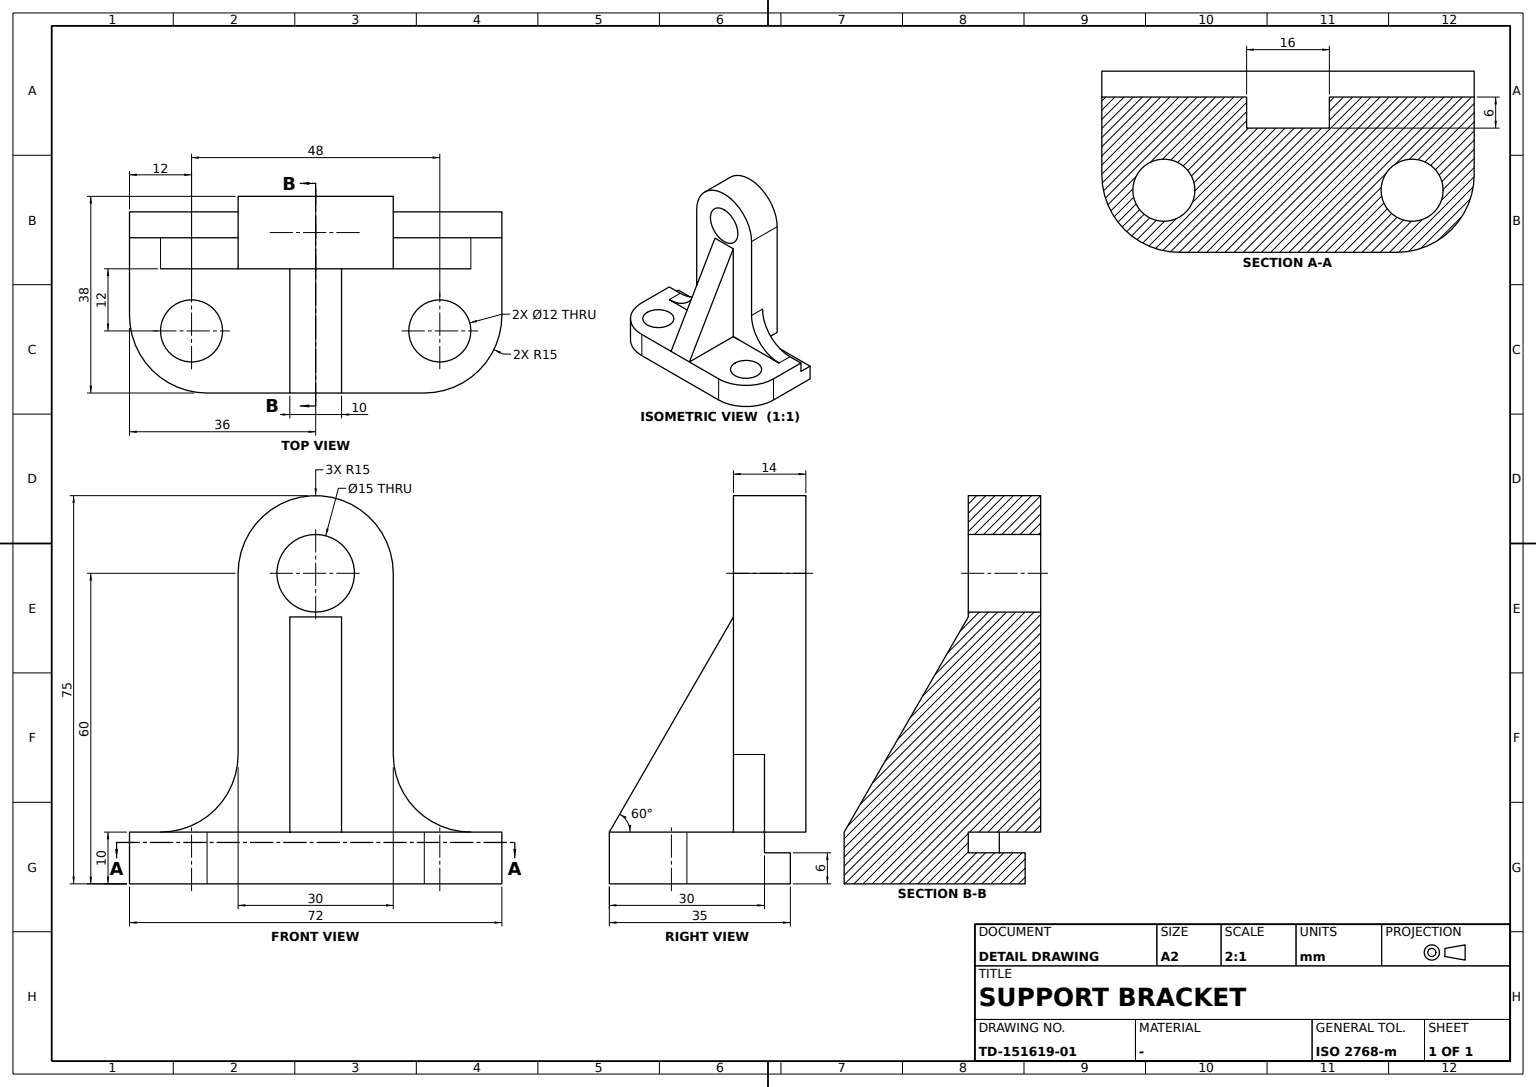
ISO-10303-21;
HEADER;
FILE_DESCRIPTION((''),'2;1');
FILE_NAME('','',(''),(''),'','','');
FILE_SCHEMA(('AUTOMOTIVE_DESIGN'));
ENDSEC;
DATA;
#1=APPLICATION_CONTEXT('');
#2=PRODUCT_CONTEXT('',#1,'mechanical');
#3=PRODUCT('','','',(#2));
#4=PRODUCT_DEFINITION_FORMATION('','',#3);
#5=PRODUCT_DEFINITION_CONTEXT('',#1,'design');
#6=PRODUCT_DEFINITION('','',#4,#5);
#7=PRODUCT_DEFINITION_SHAPE('','',#6);
#8=(LENGTH_UNIT()NAMED_UNIT(*)SI_UNIT(.MILLI.,.METRE.));
#9=(NAMED_UNIT(*)PLANE_ANGLE_UNIT()SI_UNIT($,.RADIAN.));
#10=(NAMED_UNIT(*)SI_UNIT($,.STERADIAN.)SOLID_ANGLE_UNIT());
#11=UNCERTAINTY_MEASURE_WITH_UNIT(LENGTH_MEASURE(0.005),#8,'distance_accuracy_value','');
#12=(GEOMETRIC_REPRESENTATION_CONTEXT(3)GLOBAL_UNCERTAINTY_ASSIGNED_CONTEXT((#11))GLOBAL_UNIT_ASSIGNED_CONTEXT((#8,#9,#10))REPRESENTATION_CONTEXT('',''));
#13=CARTESIAN_POINT('',(30.,6.5,5.));
#14=VERTEX_POINT('',#13);
#15=CARTESIAN_POINT('',(15.,6.5,20.));
#16=VERTEX_POINT('',#15);
#17=CARTESIAN_POINT('',(30.,6.5,20.));
#18=DIRECTION('',(0.,1.,0.));
#19=DIRECTION('',(0.,0.,1.));
#20=AXIS2_PLACEMENT_3D('',#17,#18,#19);
#21=CIRCLE('',#20,15.);
#22=EDGE_CURVE('',#14,#16,#21,.T.);
#23=ORIENTED_EDGE('',*,*,#22,.F.);
#24=CARTESIAN_POINT('',(30.,12.5,5.));
#25=VERTEX_POINT('',#24);
#26=CARTESIAN_POINT('',(30.,-0.1,5.));
#27=VECTOR('',#18,1000.);
#28=LINE('',#26,#27);
#29=EDGE_CURVE('',#14,#25,#28,.T.);
#30=ORIENTED_EDGE('',*,*,#29,.T.);
#31=CARTESIAN_POINT('',(15.,12.5,20.));
#32=VERTEX_POINT('',#31);
#33=CARTESIAN_POINT('',(30.,12.5,20.));
#34=DIRECTION('',(0.,-1.,0.));
#35=DIRECTION('',(0.,0.,-1.));
#36=AXIS2_PLACEMENT_3D('',#33,#34,#35);
#37=CIRCLE('',#36,15.);
#38=EDGE_CURVE('',#32,#25,#37,.T.);
#39=ORIENTED_EDGE('',*,*,#38,.F.);
#40=CARTESIAN_POINT('',(15.,-0.1,20.));
#41=LINE('',#40,#27);
#42=EDGE_CURVE('',#16,#32,#41,.T.);
#43=ORIENTED_EDGE('',*,*,#42,.F.);
#44=EDGE_LOOP('',(#23,#30,#39,#43));
#45=FACE_BOUND('',#44,.T.);
#46=CARTESIAN_POINT('',(30.,-0.1,20.));
#47=AXIS2_PLACEMENT_3D('',#46,#18,#35);
#48=CYLINDRICAL_SURFACE('',#47,15.);
#49=ADVANCED_FACE('',(#45),#48,.F.);
#50=CARTESIAN_POINT('',(-5.,6.5,46.569219));
#51=VERTEX_POINT('',#50);
#52=CARTESIAN_POINT('',(-5.,6.5,5.));
#53=VERTEX_POINT('',#52);
#54=CARTESIAN_POINT('',(-5.,6.5,0.));
#55=VECTOR('',#35,1000.);
#56=LINE('',#54,#55);
#57=EDGE_CURVE('',#51,#53,#56,.T.);
#58=ORIENTED_EDGE('',*,*,#57,.T.);
#59=CARTESIAN_POINT('',(-5.,-17.5,5.));
#60=VERTEX_POINT('',#59);
#61=CARTESIAN_POINT('',(-5.,0.,5.));
#62=LINE('',#61,#27);
#63=EDGE_CURVE('',#60,#53,#62,.T.);
#64=ORIENTED_EDGE('',*,*,#63,.F.);
#65=CARTESIAN_POINT('',(-5.,-15.290064,8.827722));
#66=DIRECTION('',(0.,0.5,0.866025404));
#67=VECTOR('',#66,1000.);
#68=LINE('',#65,#67);
#69=EDGE_CURVE('',#60,#51,#68,.T.);
#70=ORIENTED_EDGE('',*,*,#69,.T.);
#71=EDGE_LOOP('',(#58,#64,#70));
#72=FACE_BOUND('',#71,.T.);
#73=CARTESIAN_POINT('',(-5.,0.,0.));
#74=DIRECTION('',(1.,0.,0.));
#75=AXIS2_PLACEMENT_3D('',#73,#74,#18);
#76=PLANE('',#75);
#77=ADVANCED_FACE('',(#72),#76,.F.);
#78=CARTESIAN_POINT('',(-21.,-17.5,5.));
#79=VERTEX_POINT('',#78);
#80=CARTESIAN_POINT('',(-36.,-2.5,5.));
#81=VERTEX_POINT('',#80);
#82=CARTESIAN_POINT('',(-21.,-2.5,5.));
#83=DIRECTION('',(-1.,0.,0.));
#84=AXIS2_PLACEMENT_3D('',#82,#35,#83);
#85=CIRCLE('',#84,15.);
#86=EDGE_CURVE('',#79,#81,#85,.T.);
#87=ORIENTED_EDGE('',*,*,#86,.T.);
#88=CARTESIAN_POINT('',(-36.,-2.5,-5.));
#89=VERTEX_POINT('',#88);
#90=CARTESIAN_POINT('',(-36.,-2.5,0.));
#91=VECTOR('',#19,1000.);
#92=LINE('',#90,#91);
#93=EDGE_CURVE('',#89,#81,#92,.T.);
#94=ORIENTED_EDGE('',*,*,#93,.F.);
#95=CARTESIAN_POINT('',(-21.,-17.5,-5.));
#96=VERTEX_POINT('',#95);
#97=CARTESIAN_POINT('',(-21.,-2.5,-5.));
#98=AXIS2_PLACEMENT_3D('',#97,#19,#74);
#99=CIRCLE('',#98,15.);
#100=EDGE_CURVE('',#89,#96,#99,.T.);
#101=ORIENTED_EDGE('',*,*,#100,.T.);
#102=CARTESIAN_POINT('',(-21.,-17.5,0.));
#103=LINE('',#102,#91);
#104=EDGE_CURVE('',#96,#79,#103,.T.);
#105=ORIENTED_EDGE('',*,*,#104,.T.);
#106=EDGE_LOOP('',(#87,#94,#101,#105));
#107=FACE_BOUND('',#106,.T.);
#108=CARTESIAN_POINT('',(-21.,-2.5,0.));
#109=AXIS2_PLACEMENT_3D('',#108,#19,#83);
#110=CYLINDRICAL_SURFACE('',#109,15.);
#111=ADVANCED_FACE('',(#107),#110,.T.);
#112=CARTESIAN_POINT('',(15.,6.5,55.));
#113=VERTEX_POINT('',#112);
#114=CARTESIAN_POINT('',(15.,20.5,55.));
#115=VERTEX_POINT('',#114);
#116=CARTESIAN_POINT('',(15.,13.5,55.));
#117=LINE('',#116,#27);
#118=EDGE_CURVE('',#113,#115,#117,.T.);
#119=ORIENTED_EDGE('',*,*,#118,.F.);
#120=CARTESIAN_POINT('',(15.,6.5,0.));
#121=LINE('',#120,#55);
#122=EDGE_CURVE('',#113,#16,#121,.T.);
#123=ORIENTED_EDGE('',*,*,#122,.T.);
#124=ORIENTED_EDGE('',*,*,#42,.T.);
#125=CARTESIAN_POINT('',(15.,12.5,5.));
#126=VERTEX_POINT('',#125);
#127=CARTESIAN_POINT('',(15.,12.5,55.));
#128=LINE('',#127,#55);
#129=EDGE_CURVE('',#32,#126,#128,.T.);
#130=ORIENTED_EDGE('',*,*,#129,.T.);
#131=CARTESIAN_POINT('',(15.,20.5,5.));
#132=VERTEX_POINT('',#131);
#133=CARTESIAN_POINT('',(15.,6.5,5.));
#134=LINE('',#133,#27);
#135=EDGE_CURVE('',#126,#132,#134,.T.);
#136=ORIENTED_EDGE('',*,*,#135,.T.);
#137=CARTESIAN_POINT('',(15.,20.5,0.));
#138=LINE('',#137,#55);
#139=EDGE_CURVE('',#115,#132,#138,.T.);
#140=ORIENTED_EDGE('',*,*,#139,.F.);
#141=EDGE_LOOP('',(#119,#123,#124,#130,#136,#140));
#142=FACE_BOUND('',#141,.T.);
#143=AXIS2_PLACEMENT_3D('',#112,#74,#35);
#144=PLANE('',#143);
#145=ADVANCED_FACE('',(#142),#144,.T.);
#146=CARTESIAN_POINT('',(5.,-17.5,5.));
#147=VERTEX_POINT('',#146);
#148=CARTESIAN_POINT('',(5.,6.5,5.));
#149=VERTEX_POINT('',#148);
#150=CARTESIAN_POINT('',(5.,0.,5.));
#151=LINE('',#150,#27);
#152=EDGE_CURVE('',#147,#149,#151,.T.);
#153=ORIENTED_EDGE('',*,*,#152,.T.);
#154=CARTESIAN_POINT('',(5.,6.5,46.569219));
#155=VERTEX_POINT('',#154);
#156=CARTESIAN_POINT('',(5.,6.5,0.));
#157=LINE('',#156,#55);
#158=EDGE_CURVE('',#155,#149,#157,.T.);
#159=ORIENTED_EDGE('',*,*,#158,.F.);
#160=CARTESIAN_POINT('',(5.,-15.290064,8.827722));
#161=LINE('',#160,#67);
#162=EDGE_CURVE('',#147,#155,#161,.T.);
#163=ORIENTED_EDGE('',*,*,#162,.F.);
#164=EDGE_LOOP('',(#153,#159,#163));
#165=FACE_BOUND('',#164,.T.);
#166=CARTESIAN_POINT('',(5.,0.,0.));
#167=AXIS2_PLACEMENT_3D('',#166,#74,#18);
#168=PLANE('',#167);
#169=ADVANCED_FACE('',(#165),#168,.T.);
#170=ORIENTED_EDGE('',*,*,#139,.T.);
#171=CARTESIAN_POINT('',(-15.,20.5,5.));
#172=VERTEX_POINT('',#171);
#173=CARTESIAN_POINT('',(0.,20.5,5.));
#174=VECTOR('',#83,1000.);
#175=LINE('',#173,#174);
#176=EDGE_CURVE('',#132,#172,#175,.T.);
#177=ORIENTED_EDGE('',*,*,#176,.T.);
#178=CARTESIAN_POINT('',(-15.,20.5,55.));
#179=VERTEX_POINT('',#178);
#180=CARTESIAN_POINT('',(-15.,20.5,0.));
#181=LINE('',#180,#91);
#182=EDGE_CURVE('',#172,#179,#181,.T.);
#183=ORIENTED_EDGE('',*,*,#182,.T.);
#184=CARTESIAN_POINT('',(0.,20.5,55.));
#185=AXIS2_PLACEMENT_3D('',#184,#18,#19);
#186=CIRCLE('',#185,15.);
#187=EDGE_CURVE('',#179,#115,#186,.T.);
#188=ORIENTED_EDGE('',*,*,#187,.T.);
#189=EDGE_LOOP('',(#170,#177,#183,#188));
#190=FACE_BOUND('',#189,.T.);
#191=CARTESIAN_POINT('',(0.,20.5,62.5));
#192=VERTEX_POINT('',#191);
#193=CIRCLE('',#185,7.5);
#194=EDGE_CURVE('',#192,#192,#193,.T.);
#195=ORIENTED_EDGE('',*,*,#194,.F.);
#196=EDGE_LOOP('',(#195));
#197=FACE_BOUND('',#196,.T.);
#198=CARTESIAN_POINT('',(0.,20.5,0.));
#199=AXIS2_PLACEMENT_3D('',#198,#18,#83);
#200=PLANE('',#199);
#201=ADVANCED_FACE('',(#190,#197),#200,.T.);
#202=CARTESIAN_POINT('',(-18.,-5.5,-5.));
#203=VERTEX_POINT('',#202);
#204=CARTESIAN_POINT('',(-24.,-5.5,-5.));
#205=AXIS2_PLACEMENT_3D('',#204,#19,#74);
#206=CIRCLE('',#205,6.);
#207=EDGE_CURVE('',#203,#203,#206,.T.);
#208=ORIENTED_EDGE('',*,*,#207,.F.);
#209=EDGE_LOOP('',(#208));
#210=FACE_BOUND('',#209,.T.);
#211=CARTESIAN_POINT('',(-30.,-5.5,5.));
#212=VERTEX_POINT('',#211);
#213=CARTESIAN_POINT('',(-24.,-5.5,5.));
#214=AXIS2_PLACEMENT_3D('',#213,#35,#83);
#215=CIRCLE('',#214,6.);
#216=EDGE_CURVE('',#212,#212,#215,.F.);
#217=ORIENTED_EDGE('',*,*,#216,.T.);
#218=EDGE_LOOP('',(#217));
#219=FACE_BOUND('',#218,.T.);
#220=CARTESIAN_POINT('',(-24.,-5.5,-0.66));
#221=AXIS2_PLACEMENT_3D('',#220,#19,#34);
#222=CYLINDRICAL_SURFACE('',#221,6.);
#223=ADVANCED_FACE('',(#210,#219),#222,.F.);
#224=ORIENTED_EDGE('',*,*,#187,.F.);
#225=CARTESIAN_POINT('',(-15.,6.5,55.));
#226=VERTEX_POINT('',#225);
#227=CARTESIAN_POINT('',(-15.,13.5,55.));
#228=LINE('',#227,#27);
#229=EDGE_CURVE('',#226,#179,#228,.T.);
#230=ORIENTED_EDGE('',*,*,#229,.F.);
#231=CARTESIAN_POINT('',(0.,6.5,55.));
#232=AXIS2_PLACEMENT_3D('',#231,#18,#19);
#233=CIRCLE('',#232,15.);
#234=EDGE_CURVE('',#226,#113,#233,.T.);
#235=ORIENTED_EDGE('',*,*,#234,.T.);
#236=ORIENTED_EDGE('',*,*,#118,.T.);
#237=EDGE_LOOP('',(#224,#230,#235,#236));
#238=FACE_BOUND('',#237,.T.);
#239=CARTESIAN_POINT('',(0.,13.5,55.));
#240=AXIS2_PLACEMENT_3D('',#239,#18,#83);
#241=CYLINDRICAL_SURFACE('',#240,15.);
#242=ADVANCED_FACE('',(#238),#241,.T.);
#243=CARTESIAN_POINT('',(8.,6.5,1.));
#244=VERTEX_POINT('',#243);
#245=CARTESIAN_POINT('',(-8.,6.5,1.));
#246=VERTEX_POINT('',#245);
#247=CARTESIAN_POINT('',(0.,6.5,1.));
#248=LINE('',#247,#174);
#249=EDGE_CURVE('',#244,#246,#248,.T.);
#250=ORIENTED_EDGE('',*,*,#249,.T.);
#251=CARTESIAN_POINT('',(-8.,6.5,5.));
#252=VERTEX_POINT('',#251);
#253=LINE('',#245,#91);
#254=EDGE_CURVE('',#246,#252,#253,.T.);
#255=ORIENTED_EDGE('',*,*,#254,.T.);
#256=CARTESIAN_POINT('',(0.,6.5,5.));
#257=LINE('',#256,#174);
#258=EDGE_CURVE('',#149,#252,#257,.T.);
#259=ORIENTED_EDGE('',*,*,#258,.F.);
#260=CARTESIAN_POINT('',(8.,6.5,5.));
#261=VERTEX_POINT('',#260);
#262=EDGE_CURVE('',#261,#149,#257,.T.);
#263=ORIENTED_EDGE('',*,*,#262,.F.);
#264=LINE('',#260,#55);
#265=EDGE_CURVE('',#261,#244,#264,.T.);
#266=ORIENTED_EDGE('',*,*,#265,.T.);
#267=EDGE_LOOP('',(#250,#255,#259,#263,#266));
#268=FACE_BOUND('',#267,.T.);
#269=CARTESIAN_POINT('',(0.,6.5,0.));
#270=AXIS2_PLACEMENT_3D('',#269,#18,#83);
#271=PLANE('',#270);
#272=ADVANCED_FACE('',(#268),#271,.T.);
#273=CARTESIAN_POINT('',(36.,-2.5,5.));
#274=VERTEX_POINT('',#273);
#275=CARTESIAN_POINT('',(36.,12.5,5.));
#276=VERTEX_POINT('',#275);
#277=CARTESIAN_POINT('',(36.,0.,5.));
#278=LINE('',#277,#27);
#279=EDGE_CURVE('',#274,#276,#278,.T.);
#280=ORIENTED_EDGE('',*,*,#279,.T.);
#281=CARTESIAN_POINT('',(0.,12.5,5.));
#282=VECTOR('',#74,1000.);
#283=LINE('',#281,#282);
#284=EDGE_CURVE('',#25,#276,#283,.T.);
#285=ORIENTED_EDGE('',*,*,#284,.F.);
#286=ORIENTED_EDGE('',*,*,#29,.F.);
#287=EDGE_CURVE('',#14,#261,#257,.T.);
#288=ORIENTED_EDGE('',*,*,#287,.T.);
#289=ORIENTED_EDGE('',*,*,#262,.T.);
#290=ORIENTED_EDGE('',*,*,#152,.F.);
#291=CARTESIAN_POINT('',(21.,-17.5,5.));
#292=VERTEX_POINT('',#291);
#293=CARTESIAN_POINT('',(0.,-17.5,5.));
#294=LINE('',#293,#282);
#295=EDGE_CURVE('',#147,#292,#294,.T.);
#296=ORIENTED_EDGE('',*,*,#295,.T.);
#297=CARTESIAN_POINT('',(21.,-2.5,5.));
#298=AXIS2_PLACEMENT_3D('',#297,#35,#83);
#299=CIRCLE('',#298,15.);
#300=EDGE_CURVE('',#274,#292,#299,.T.);
#301=ORIENTED_EDGE('',*,*,#300,.F.);
#302=EDGE_LOOP('',(#280,#285,#286,#288,#289,#290,#296,#301));
#303=FACE_BOUND('',#302,.T.);
#304=CARTESIAN_POINT('',(18.,-5.5,5.));
#305=VERTEX_POINT('',#304);
#306=CARTESIAN_POINT('',(24.,-5.5,5.));
#307=AXIS2_PLACEMENT_3D('',#306,#35,#83);
#308=CIRCLE('',#307,6.);
#309=EDGE_CURVE('',#305,#305,#308,.F.);
#310=ORIENTED_EDGE('',*,*,#309,.F.);
#311=EDGE_LOOP('',(#310));
#312=FACE_BOUND('',#311,.T.);
#313=AXIS2_PLACEMENT_3D('',#293,#35,#18);
#314=PLANE('',#313);
#315=ADVANCED_FACE('',(#303,#312),#314,.F.);
#316=CARTESIAN_POINT('',(8.,12.5,1.));
#317=VERTEX_POINT('',#316);
#318=VECTOR('',#34,1000.);
#319=LINE('',#316,#318);
#320=EDGE_CURVE('',#317,#244,#319,.T.);
#321=ORIENTED_EDGE('',*,*,#320,.T.);
#322=ORIENTED_EDGE('',*,*,#265,.F.);
#323=CARTESIAN_POINT('',(8.,12.5,5.));
#324=VERTEX_POINT('',#323);
#325=LINE('',#323,#318);
#326=EDGE_CURVE('',#324,#261,#325,.T.);
#327=ORIENTED_EDGE('',*,*,#326,.F.);
#328=LINE('',#323,#55);
#329=EDGE_CURVE('',#324,#317,#328,.T.);
#330=ORIENTED_EDGE('',*,*,#329,.T.);
#331=EDGE_LOOP('',(#321,#322,#327,#330));
#332=FACE_BOUND('',#331,.T.);
#333=AXIS2_PLACEMENT_3D('',#323,#83,#35);
#334=PLANE('',#333);
#335=ADVANCED_FACE('',(#332),#334,.T.);
#336=ORIENTED_EDGE('',*,*,#194,.T.);
#337=EDGE_LOOP('',(#336));
#338=FACE_BOUND('',#337,.T.);
#339=CARTESIAN_POINT('',(0.,6.5,62.5));
#340=VERTEX_POINT('',#339);
#341=CIRCLE('',#232,7.5);
#342=EDGE_CURVE('',#340,#340,#341,.T.);
#343=ORIENTED_EDGE('',*,*,#342,.F.);
#344=EDGE_LOOP('',(#343));
#345=FACE_BOUND('',#344,.T.);
#346=CYLINDRICAL_SURFACE('',#240,7.5);
#347=ADVANCED_FACE('',(#338,#345),#346,.F.);
#348=CARTESIAN_POINT('',(-8.,12.5,1.));
#349=VERTEX_POINT('',#348);
#350=LINE('',#348,#318);
#351=EDGE_CURVE('',#349,#246,#350,.T.);
#352=ORIENTED_EDGE('',*,*,#351,.T.);
#353=ORIENTED_EDGE('',*,*,#249,.F.);
#354=ORIENTED_EDGE('',*,*,#320,.F.);
#355=CARTESIAN_POINT('',(36.,12.5,1.));
#356=VERTEX_POINT('',#355);
#357=CARTESIAN_POINT('',(0.,12.5,1.));
#358=LINE('',#357,#282);
#359=EDGE_CURVE('',#317,#356,#358,.T.);
#360=ORIENTED_EDGE('',*,*,#359,.T.);
#361=CARTESIAN_POINT('',(36.,17.5,1.));
#362=VERTEX_POINT('',#361);
#363=CARTESIAN_POINT('',(36.,0.,1.));
#364=LINE('',#363,#27);
#365=EDGE_CURVE('',#356,#362,#364,.T.);
#366=ORIENTED_EDGE('',*,*,#365,.T.);
#367=CARTESIAN_POINT('',(-36.,17.5,1.));
#368=VERTEX_POINT('',#367);
#369=CARTESIAN_POINT('',(0.,17.5,1.));
#370=LINE('',#369,#282);
#371=EDGE_CURVE('',#368,#362,#370,.T.);
#372=ORIENTED_EDGE('',*,*,#371,.F.);
#373=CARTESIAN_POINT('',(-36.,12.5,1.));
#374=VERTEX_POINT('',#373);
#375=CARTESIAN_POINT('',(-36.,0.,1.));
#376=LINE('',#375,#27);
#377=EDGE_CURVE('',#374,#368,#376,.T.);
#378=ORIENTED_EDGE('',*,*,#377,.F.);
#379=EDGE_CURVE('',#374,#349,#358,.T.);
#380=ORIENTED_EDGE('',*,*,#379,.T.);
#381=EDGE_LOOP('',(#352,#353,#354,#360,#366,#372,#378,#380));
#382=FACE_BOUND('',#381,.T.);
#383=AXIS2_PLACEMENT_3D('',#357,#35,#18);
#384=PLANE('',#383);
#385=ADVANCED_FACE('',(#382),#384,.F.);
#386=CARTESIAN_POINT('',(30.,-5.5,-5.));
#387=VERTEX_POINT('',#386);
#388=CARTESIAN_POINT('',(24.,-5.5,-5.));
#389=AXIS2_PLACEMENT_3D('',#388,#19,#74);
#390=CIRCLE('',#389,6.);
#391=EDGE_CURVE('',#387,#387,#390,.T.);
#392=ORIENTED_EDGE('',*,*,#391,.F.);
#393=EDGE_LOOP('',(#392));
#394=FACE_BOUND('',#393,.T.);
#395=ORIENTED_EDGE('',*,*,#309,.T.);
#396=EDGE_LOOP('',(#395));
#397=FACE_BOUND('',#396,.T.);
#398=CARTESIAN_POINT('',(24.,-5.5,-0.66));
#399=AXIS2_PLACEMENT_3D('',#398,#19,#34);
#400=CYLINDRICAL_SURFACE('',#399,6.);
#401=ADVANCED_FACE('',(#394,#397),#400,.F.);
#402=ORIENTED_EDGE('',*,*,#229,.T.);
#403=ORIENTED_EDGE('',*,*,#182,.F.);
#404=CARTESIAN_POINT('',(-15.,12.5,5.));
#405=VERTEX_POINT('',#404);
#406=CARTESIAN_POINT('',(-15.,-17.5,5.));
#407=LINE('',#406,#27);
#408=EDGE_CURVE('',#405,#172,#407,.T.);
#409=ORIENTED_EDGE('',*,*,#408,.F.);
#410=CARTESIAN_POINT('',(-15.,12.5,20.));
#411=VERTEX_POINT('',#410);
#412=LINE('',#404,#91);
#413=EDGE_CURVE('',#405,#411,#412,.T.);
#414=ORIENTED_EDGE('',*,*,#413,.T.);
#415=CARTESIAN_POINT('',(-15.,6.5,20.));
#416=VERTEX_POINT('',#415);
#417=CARTESIAN_POINT('',(-15.,-0.1,20.));
#418=LINE('',#417,#318);
#419=EDGE_CURVE('',#411,#416,#418,.T.);
#420=ORIENTED_EDGE('',*,*,#419,.T.);
#421=CARTESIAN_POINT('',(-15.,6.5,0.));
#422=LINE('',#421,#91);
#423=EDGE_CURVE('',#416,#226,#422,.T.);
#424=ORIENTED_EDGE('',*,*,#423,.T.);
#425=EDGE_LOOP('',(#402,#403,#409,#414,#420,#424));
#426=FACE_BOUND('',#425,.T.);
#427=CARTESIAN_POINT('',(-15.,6.5,5.));
#428=AXIS2_PLACEMENT_3D('',#427,#83,#19);
#429=PLANE('',#428);
#430=ADVANCED_FACE('',(#426),#429,.T.);
#431=ORIENTED_EDGE('',*,*,#162,.T.);
#432=CARTESIAN_POINT('',(0.,6.5,46.569219));
#433=LINE('',#432,#282);
#434=EDGE_CURVE('',#51,#155,#433,.T.);
#435=ORIENTED_EDGE('',*,*,#434,.F.);
#436=ORIENTED_EDGE('',*,*,#69,.F.);
#437=EDGE_CURVE('',#60,#147,#294,.T.);
#438=ORIENTED_EDGE('',*,*,#437,.T.);
#439=EDGE_LOOP('',(#431,#435,#436,#438));
#440=FACE_BOUND('',#439,.T.);
#441=DIRECTION('',(0.,0.866025404,-0.5));
#442=AXIS2_PLACEMENT_3D('',#293,#441,#66);
#443=PLANE('',#442);
#444=ADVANCED_FACE('',(#440),#443,.F.);
#445=ORIENTED_EDGE('',*,*,#300,.T.);
#446=CARTESIAN_POINT('',(21.,-17.5,-5.));
#447=VERTEX_POINT('',#446);
#448=CARTESIAN_POINT('',(21.,-17.5,0.));
#449=LINE('',#448,#91);
#450=EDGE_CURVE('',#447,#292,#449,.T.);
#451=ORIENTED_EDGE('',*,*,#450,.F.);
#452=CARTESIAN_POINT('',(36.,-2.5,-5.));
#453=VERTEX_POINT('',#452);
#454=CARTESIAN_POINT('',(21.,-2.5,-5.));
#455=AXIS2_PLACEMENT_3D('',#454,#19,#74);
#456=CIRCLE('',#455,15.);
#457=EDGE_CURVE('',#447,#453,#456,.T.);
#458=ORIENTED_EDGE('',*,*,#457,.T.);
#459=CARTESIAN_POINT('',(36.,-2.5,0.));
#460=LINE('',#459,#91);
#461=EDGE_CURVE('',#453,#274,#460,.T.);
#462=ORIENTED_EDGE('',*,*,#461,.T.);
#463=EDGE_LOOP('',(#445,#451,#458,#462));
#464=FACE_BOUND('',#463,.T.);
#465=CARTESIAN_POINT('',(21.,-2.5,0.));
#466=AXIS2_PLACEMENT_3D('',#465,#19,#34);
#467=CYLINDRICAL_SURFACE('',#466,15.);
#468=ADVANCED_FACE('',(#464),#467,.T.);
#469=ORIENTED_EDGE('',*,*,#329,.F.);
#470=EDGE_CURVE('',#324,#126,#283,.T.);
#471=ORIENTED_EDGE('',*,*,#470,.T.);
#472=ORIENTED_EDGE('',*,*,#129,.F.);
#473=ORIENTED_EDGE('',*,*,#38,.T.);
#474=ORIENTED_EDGE('',*,*,#284,.T.);
#475=CARTESIAN_POINT('',(36.,12.5,0.));
#476=LINE('',#475,#55);
#477=EDGE_CURVE('',#276,#356,#476,.T.);
#478=ORIENTED_EDGE('',*,*,#477,.T.);
#479=ORIENTED_EDGE('',*,*,#359,.F.);
#480=EDGE_LOOP('',(#469,#471,#472,#473,#474,#478,#479));
#481=FACE_BOUND('',#480,.T.);
#482=AXIS2_PLACEMENT_3D('',#281,#34,#35);
#483=PLANE('',#482);
#484=ADVANCED_FACE('',(#481),#483,.F.);
#485=ORIENTED_EDGE('',*,*,#461,.F.);
#486=CARTESIAN_POINT('',(36.,17.5,-5.));
#487=VERTEX_POINT('',#486);
#488=CARTESIAN_POINT('',(36.,0.,-5.));
#489=LINE('',#488,#318);
#490=EDGE_CURVE('',#487,#453,#489,.T.);
#491=ORIENTED_EDGE('',*,*,#490,.F.);
#492=CARTESIAN_POINT('',(36.,17.5,0.));
#493=LINE('',#492,#55);
#494=EDGE_CURVE('',#362,#487,#493,.T.);
#495=ORIENTED_EDGE('',*,*,#494,.F.);
#496=ORIENTED_EDGE('',*,*,#365,.F.);
#497=ORIENTED_EDGE('',*,*,#477,.F.);
#498=ORIENTED_EDGE('',*,*,#279,.F.);
#499=EDGE_LOOP('',(#485,#491,#495,#496,#497,#498));
#500=FACE_BOUND('',#499,.T.);
#501=CARTESIAN_POINT('',(36.,0.,0.));
#502=AXIS2_PLACEMENT_3D('',#501,#74,#18);
#503=PLANE('',#502);
#504=ADVANCED_FACE('',(#500),#503,.T.);
#505=CARTESIAN_POINT('',(-36.,17.5,-5.));
#506=VERTEX_POINT('',#505);
#507=CARTESIAN_POINT('',(-36.,0.,-5.));
#508=LINE('',#507,#318);
#509=EDGE_CURVE('',#506,#89,#508,.T.);
#510=ORIENTED_EDGE('',*,*,#509,.T.);
#511=ORIENTED_EDGE('',*,*,#93,.T.);
#512=CARTESIAN_POINT('',(-36.,12.5,5.));
#513=VERTEX_POINT('',#512);
#514=CARTESIAN_POINT('',(-36.,0.,5.));
#515=LINE('',#514,#27);
#516=EDGE_CURVE('',#81,#513,#515,.T.);
#517=ORIENTED_EDGE('',*,*,#516,.T.);
#518=CARTESIAN_POINT('',(-36.,12.5,0.));
#519=LINE('',#518,#55);
#520=EDGE_CURVE('',#513,#374,#519,.T.);
#521=ORIENTED_EDGE('',*,*,#520,.T.);
#522=ORIENTED_EDGE('',*,*,#377,.T.);
#523=CARTESIAN_POINT('',(-36.,17.5,0.));
#524=LINE('',#523,#55);
#525=EDGE_CURVE('',#368,#506,#524,.T.);
#526=ORIENTED_EDGE('',*,*,#525,.T.);
#527=EDGE_LOOP('',(#510,#511,#517,#521,#522,#526));
#528=FACE_BOUND('',#527,.T.);
#529=CARTESIAN_POINT('',(-36.,0.,0.));
#530=AXIS2_PLACEMENT_3D('',#529,#74,#18);
#531=PLANE('',#530);
#532=ADVANCED_FACE('',(#528),#531,.F.);
#533=ORIENTED_EDGE('',*,*,#494,.T.);
#534=CARTESIAN_POINT('',(0.,17.5,-5.));
#535=LINE('',#534,#282);
#536=EDGE_CURVE('',#506,#487,#535,.T.);
#537=ORIENTED_EDGE('',*,*,#536,.F.);
#538=ORIENTED_EDGE('',*,*,#525,.F.);
#539=ORIENTED_EDGE('',*,*,#371,.T.);
#540=EDGE_LOOP('',(#533,#537,#538,#539));
#541=FACE_BOUND('',#540,.T.);
#542=AXIS2_PLACEMENT_3D('',#369,#34,#35);
#543=PLANE('',#542);
#544=ADVANCED_FACE('',(#541),#543,.F.);
#545=ORIENTED_EDGE('',*,*,#86,.F.);
#546=EDGE_CURVE('',#79,#60,#294,.T.);
#547=ORIENTED_EDGE('',*,*,#546,.T.);
#548=ORIENTED_EDGE('',*,*,#63,.T.);
#549=CARTESIAN_POINT('',(-30.,6.5,5.));
#550=VERTEX_POINT('',#549);
#551=EDGE_CURVE('',#53,#550,#257,.T.);
#552=ORIENTED_EDGE('',*,*,#551,.T.);
#553=CARTESIAN_POINT('',(-30.,12.5,5.));
#554=VERTEX_POINT('',#553);
#555=CARTESIAN_POINT('',(-30.,-0.1,5.));
#556=LINE('',#555,#318);
#557=EDGE_CURVE('',#554,#550,#556,.T.);
#558=ORIENTED_EDGE('',*,*,#557,.F.);
#559=EDGE_CURVE('',#513,#554,#283,.T.);
#560=ORIENTED_EDGE('',*,*,#559,.F.);
#561=ORIENTED_EDGE('',*,*,#516,.F.);
#562=EDGE_LOOP('',(#545,#547,#548,#552,#558,#560,#561));
#563=FACE_BOUND('',#562,.T.);
#564=ORIENTED_EDGE('',*,*,#216,.F.);
#565=EDGE_LOOP('',(#564));
#566=FACE_BOUND('',#565,.T.);
#567=ADVANCED_FACE('',(#563,#566),#314,.F.);
#568=CARTESIAN_POINT('',(-8.,12.5,5.));
#569=VERTEX_POINT('',#568);
#570=CARTESIAN_POINT('',(-8.,-17.5,5.));
#571=LINE('',#570,#318);
#572=EDGE_CURVE('',#569,#252,#571,.T.);
#573=ORIENTED_EDGE('',*,*,#572,.T.);
#574=ORIENTED_EDGE('',*,*,#254,.F.);
#575=ORIENTED_EDGE('',*,*,#351,.F.);
#576=LINE('',#568,#91);
#577=EDGE_CURVE('',#349,#569,#576,.T.);
#578=ORIENTED_EDGE('',*,*,#577,.T.);
#579=EDGE_LOOP('',(#573,#574,#575,#578));
#580=FACE_BOUND('',#579,.T.);
#581=AXIS2_PLACEMENT_3D('',#348,#74,#19);
#582=PLANE('',#581);
#583=ADVANCED_FACE('',(#580),#582,.T.);
#584=ORIENTED_EDGE('',*,*,#207,.T.);
#585=EDGE_LOOP('',(#584));
#586=FACE_BOUND('',#585,.T.);
#587=ORIENTED_EDGE('',*,*,#391,.T.);
#588=EDGE_LOOP('',(#587));
#589=FACE_BOUND('',#588,.T.);
#590=ORIENTED_EDGE('',*,*,#100,.F.);
#591=ORIENTED_EDGE('',*,*,#509,.F.);
#592=ORIENTED_EDGE('',*,*,#536,.T.);
#593=ORIENTED_EDGE('',*,*,#490,.T.);
#594=ORIENTED_EDGE('',*,*,#457,.F.);
#595=CARTESIAN_POINT('',(0.,-17.5,-5.));
#596=LINE('',#595,#282);
#597=EDGE_CURVE('',#96,#447,#596,.T.);
#598=ORIENTED_EDGE('',*,*,#597,.F.);
#599=EDGE_LOOP('',(#590,#591,#592,#593,#594,#598));
#600=FACE_BOUND('',#599,.T.);
#601=AXIS2_PLACEMENT_3D('',#534,#19,#34);
#602=PLANE('',#601);
#603=ADVANCED_FACE('',(#586,#589,#600),#602,.F.);
#604=EDGE_CURVE('',#261,#149,#257,.T.);
#605=ORIENTED_EDGE('',*,*,#604,.T.);
#606=ORIENTED_EDGE('',*,*,#258,.T.);
#607=ORIENTED_EDGE('',*,*,#572,.F.);
#608=EDGE_CURVE('',#405,#569,#283,.T.);
#609=ORIENTED_EDGE('',*,*,#608,.F.);
#610=ORIENTED_EDGE('',*,*,#408,.T.);
#611=ORIENTED_EDGE('',*,*,#176,.F.);
#612=ORIENTED_EDGE('',*,*,#135,.F.);
#613=ORIENTED_EDGE('',*,*,#470,.F.);
#614=ORIENTED_EDGE('',*,*,#326,.T.);
#615=EDGE_LOOP('',(#605,#606,#607,#609,#610,#611,#612,#613,#614));
#616=FACE_BOUND('',#615,.T.);
#617=ADVANCED_FACE('',(#616),#314,.T.);
#618=ORIENTED_EDGE('',*,*,#604,.F.);
#619=ORIENTED_EDGE('',*,*,#287,.F.);
#620=ORIENTED_EDGE('',*,*,#22,.T.);
#621=ORIENTED_EDGE('',*,*,#122,.F.);
#622=ORIENTED_EDGE('',*,*,#234,.F.);
#623=ORIENTED_EDGE('',*,*,#423,.F.);
#624=CARTESIAN_POINT('',(-30.,6.5,20.));
#625=AXIS2_PLACEMENT_3D('',#624,#18,#19);
#626=CIRCLE('',#625,15.);
#627=EDGE_CURVE('',#416,#550,#626,.T.);
#628=ORIENTED_EDGE('',*,*,#627,.T.);
#629=ORIENTED_EDGE('',*,*,#551,.F.);
#630=ORIENTED_EDGE('',*,*,#57,.F.);
#631=ORIENTED_EDGE('',*,*,#434,.T.);
#632=ORIENTED_EDGE('',*,*,#158,.T.);
#633=EDGE_LOOP('',(#618,#619,#620,#621,#622,#623,#628,#629,#630,#631,#632));
#634=FACE_BOUND('',#633,.T.);
#635=ORIENTED_EDGE('',*,*,#342,.T.);
#636=EDGE_LOOP('',(#635));
#637=FACE_BOUND('',#636,.T.);
#638=ADVANCED_FACE('',(#634,#637),#271,.F.);
#639=ORIENTED_EDGE('',*,*,#608,.T.);
#640=ORIENTED_EDGE('',*,*,#577,.F.);
#641=ORIENTED_EDGE('',*,*,#379,.F.);
#642=ORIENTED_EDGE('',*,*,#520,.F.);
#643=ORIENTED_EDGE('',*,*,#559,.T.);
#644=CARTESIAN_POINT('',(-30.,12.5,20.));
#645=AXIS2_PLACEMENT_3D('',#644,#34,#35);
#646=CIRCLE('',#645,15.);
#647=EDGE_CURVE('',#554,#411,#646,.T.);
#648=ORIENTED_EDGE('',*,*,#647,.T.);
#649=ORIENTED_EDGE('',*,*,#413,.F.);
#650=EDGE_LOOP('',(#639,#640,#641,#642,#643,#648,#649));
#651=FACE_BOUND('',#650,.T.);
#652=ADVANCED_FACE('',(#651),#483,.F.);
#653=ORIENTED_EDGE('',*,*,#647,.F.);
#654=ORIENTED_EDGE('',*,*,#557,.T.);
#655=ORIENTED_EDGE('',*,*,#627,.F.);
#656=ORIENTED_EDGE('',*,*,#419,.F.);
#657=EDGE_LOOP('',(#653,#654,#655,#656));
#658=FACE_BOUND('',#657,.T.);
#659=CARTESIAN_POINT('',(-30.,-0.1,20.));
#660=AXIS2_PLACEMENT_3D('',#659,#34,#74);
#661=CYLINDRICAL_SURFACE('',#660,15.);
#662=ADVANCED_FACE('',(#658),#661,.F.);
#663=ORIENTED_EDGE('',*,*,#295,.F.);
#664=ORIENTED_EDGE('',*,*,#437,.F.);
#665=ORIENTED_EDGE('',*,*,#546,.F.);
#666=ORIENTED_EDGE('',*,*,#104,.F.);
#667=ORIENTED_EDGE('',*,*,#597,.T.);
#668=ORIENTED_EDGE('',*,*,#450,.T.);
#669=EDGE_LOOP('',(#663,#664,#665,#666,#667,#668));
#670=FACE_BOUND('',#669,.T.);
#671=AXIS2_PLACEMENT_3D('',#595,#18,#19);
#672=PLANE('',#671);
#673=ADVANCED_FACE('',(#670),#672,.F.);
#674=CLOSED_SHELL('',(#49,#77,#111,#145,#169,#201,#223,#242,#272,#315,#335,#347,#385,#401,#430,#444,#468,#484,#504,#532,#544,#567,#583,#603,#617,#638,#652,#662,#673));
#675=MANIFOLD_SOLID_BREP('',#674);
#676=ADVANCED_BREP_SHAPE_REPRESENTATION('',(#675),#12);
#677=SHAPE_DEFINITION_REPRESENTATION(#7,#676);
ENDSEC;
END-ISO-10303-21;
